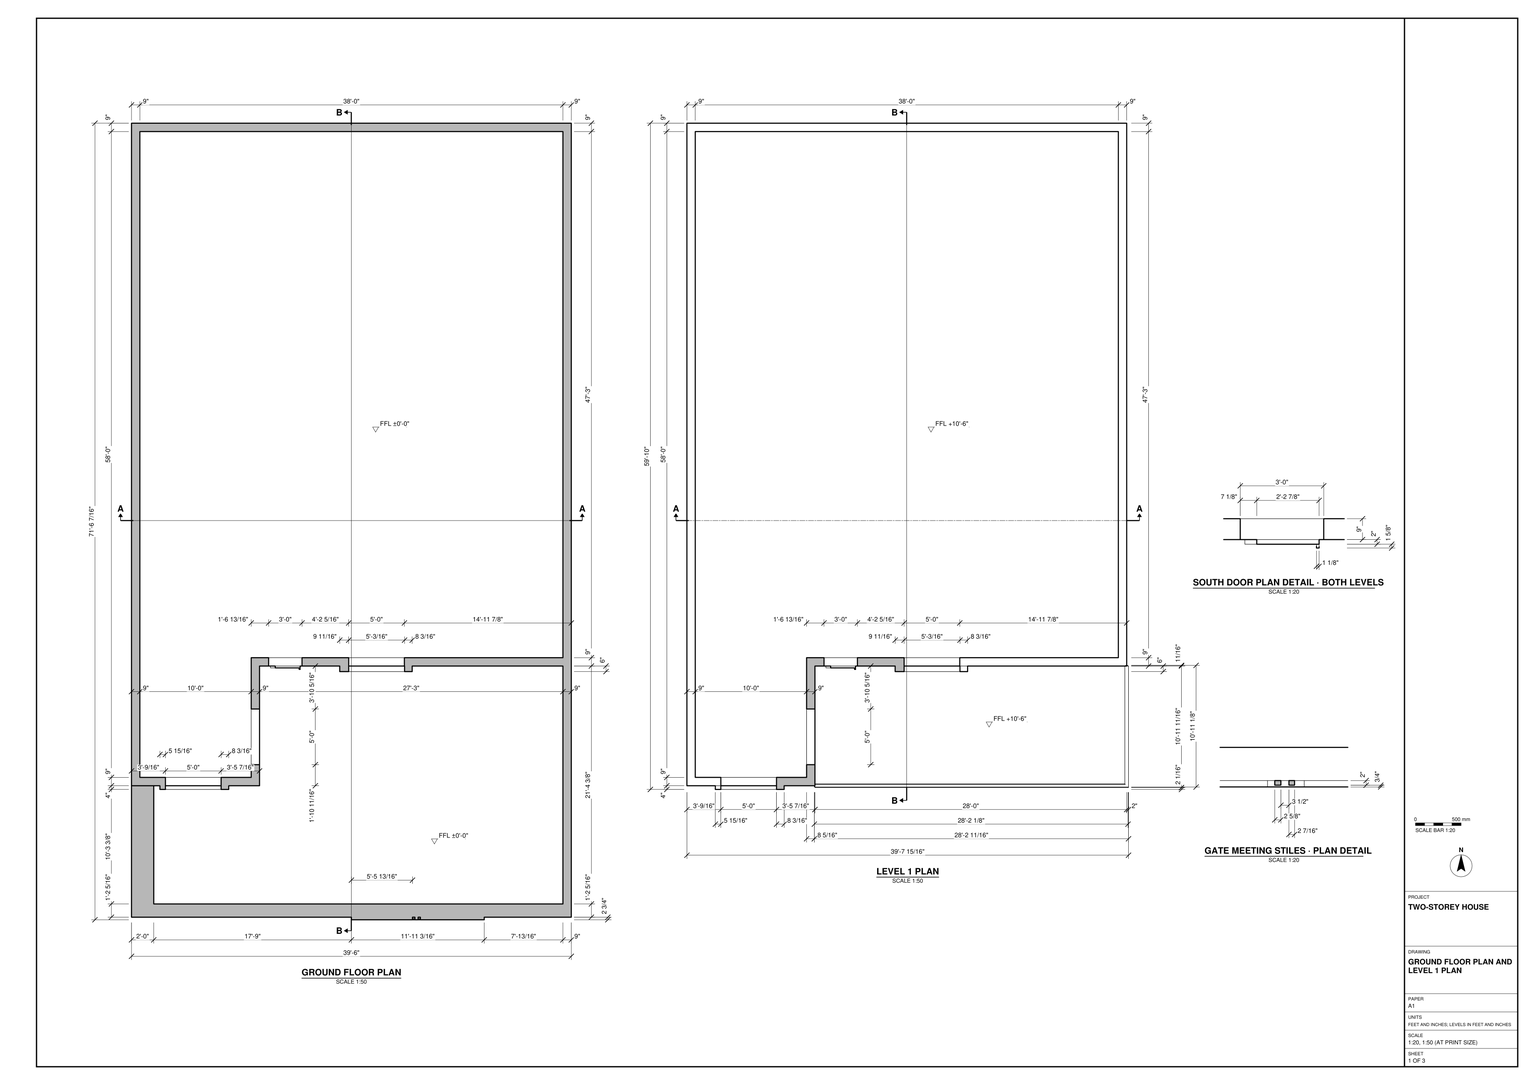
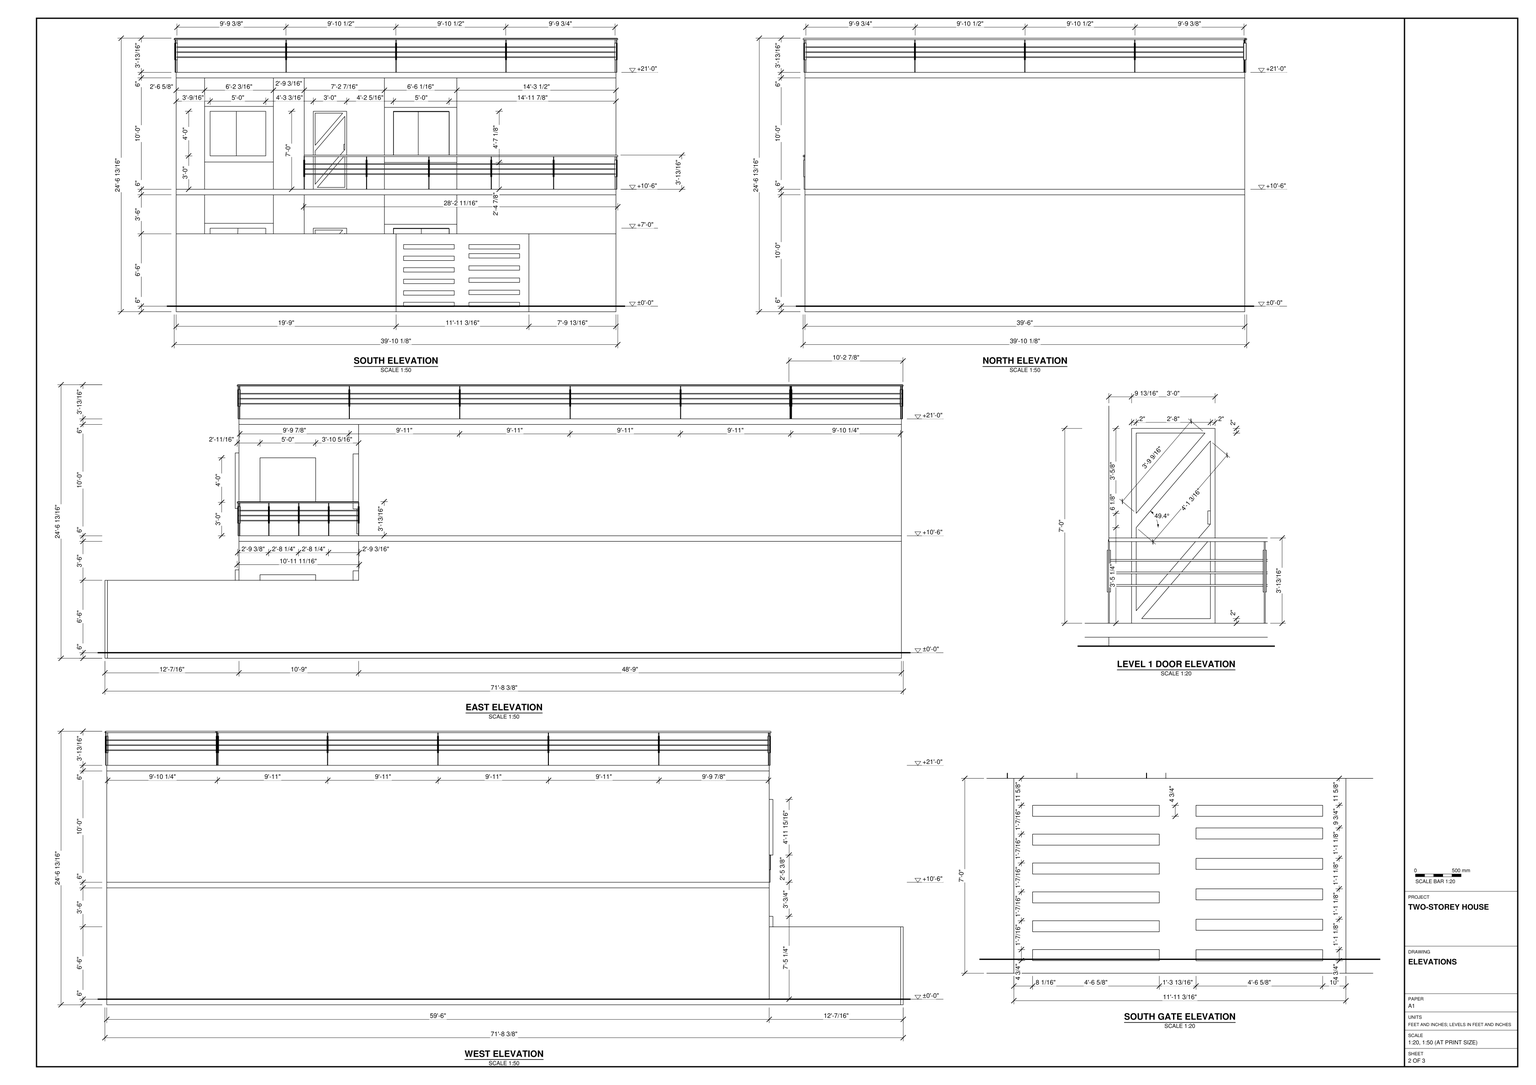
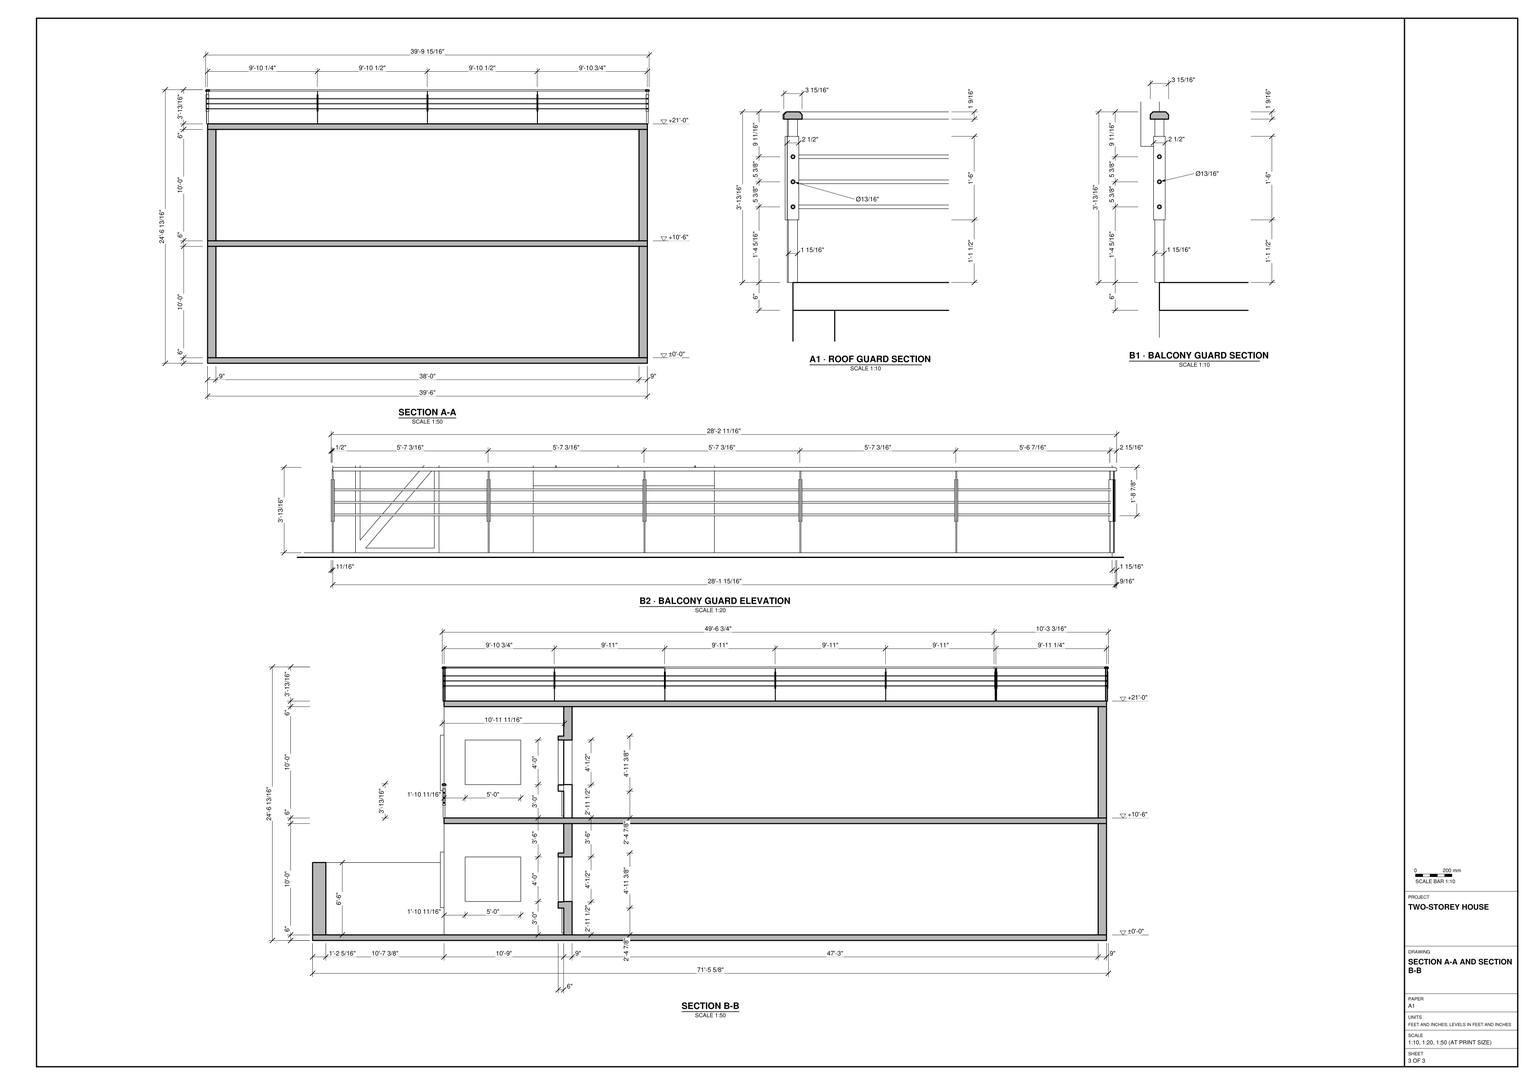
Build the house shown in task_files/diagram_01.pdf in SketchUp. Work in feet and inches. The overall model is 39'-10 3/16" wide from east to west, 71'-8 3/8" long from north to south and 24'-6 13/16" high. Set the finished floor levels at ±0'-0" and +10'-6".

Use the plans to lay out the open interior and the stepped south frontage. The west bay projects toward the forecourt, while the recessed wall beside it contains a door and a window on each floor. Follow the drawn wall thicknesses, including the 9" house walls. Use the sections to locate the ground slab, upper slab and flat roof. Extend the upper slab across the recess to form the balcony, with the roof continuing over it. Model the front and side runs of the balcony guard and the guard around the roof. Follow the details for the upper door, guard rails and posts, and the paired gate in the south forecourt wall.

Keep walls, slabs, roof, guards, gate and each furniture or joinery piece separate as groups or components. Use components for repeated parts. Any decor or loose items may be suitable library components. Save one SketchUp model as output_files/two_storey_house_with_a_balcony_and_gated_forecourt.skp.

# SketchUp Ruby script. Lengths in inches.
U = 1.inch
M = Sketchup.active_model
def pt(a) = Geom::Point3d.new(a.map { |v| v * U })
def face(e, loops, mat)
  f = e.add_face(loops[0].map { |a| pt(a) })
  loops[1..].each { |l| e.add_face(l.map { |a| pt(a) }).erase! }
  f.material = f.back_material = mat if mat
  f
end
# faces: each face lists its corners as indices into pts; further lists are holes
def faces(e, pts, list, mat = nil) = list.each { |f| face(e, (f[0].is_a?(Array) ? f : [f]).map { |l| l.map { |i| pts[i] } }, mat) }
# xy, xz, yz: faces in a plane at the given z, y or x. An outline is a flat list of corners, or four numbers for a rectangle; further outlines are holes
def ring(l) = l.size == 4 ? [[l[0], l[1]], [l[2], l[1]], [l[2], l[3]], [l[0], l[3]]] : l.each_slice(2).to_a
def flat(e, list, mat, &to3) = list.each { |f| face(e, (f[0].is_a?(Array) ? f : [f]).map { |l| ring(l).map { |u, v| to3.(u, v) } }, mat) }
def xy(e, z, list, mat = nil) = flat(e, list, mat) { |x, y| [x, y, z] }
def xz(e, y, list, mat = nil) = flat(e, list, mat) { |x, z| [x, y, z] }
def yz(e, x, list, mat = nil) = flat(e, list, mat) { |y, z| [x, y, z] }
def lines(e, pts, list) = list.each { |a, b| e.add_line(pt(pts[a]), pt(pts[b])) }
# prism: a flat outline (further loops are holes) pulled along v
def prism(e, loops, v, mat = nil)
  f = face(e, loops, mat); d = Geom::Vector3d.new(v.map { |x| x * U })
  f.pushpull(f.normal.samedirection?(d) ? d.length : -d.length)
end
def box(e, o, s, mat = nil) = prism(e, [[o, [o[0] + s[0], o[1], o[2]], [o[0] + s[0], o[1] + s[1], o[2]], [o[0], o[1] + s[1], o[2]]]], [0, 0, s[2]], mat)
def at(x, y, z, deg = 0) = Geom::Transformation.translation(pt([x, y, z])) * Geom::Transformation.rotation(ORIGIN, Z_AXIS, deg.degrees)
def axes(o, x, y, z) = Geom::Transformation.new([*x, 0, *y, 0, *z, 0, *pt(o).to_a, 1])
def part(name) = M.definitions.add(name)
# library, detail: a bought-in or finely detailed component or shape, given as its bounding box
def library(name, o, s) = part(name).tap { |d| box(d.entities, o, s) }
def detail(e, o, s) = box(e.add_group.entities, o, s)
def put(e, d, t, mat = nil) = e.add_instance(d, t).tap { |i| i.material = mat if mat }
def group(e, t, mat = nil) = e.add_group.tap { |g| g.transformation = t; g.material = mat if mat }.entities
root = M.entities
M.materials.add("Teddy_Bracelet").color = [145, 141, 147]
M.materials.add("Teddy_Shoes").color = [189, 191, 193]
M.materials.add("[Color H05]").color = [0, 255, 255]
M.materials.add("[Color M09]").color = [0, 0, 0]
M.materials.add("[Field Square Tile]").color = [217, 201, 169]
M.materials.add("[Herringbone]").color = [130, 130, 130]
M.materials.add("[Translucent Glass Blue]").color = [100, 149, 237]
M.materials["[Translucent Glass Blue]"].alpha = 0.5
M.materials.add("[Wood Board Cork]").color = [215, 201, 115]
M.materials.add("[Wood Cherry Original]").color = [152, 86, 42]
M.materials.add("[Wood Veneer 02]").color = [190, 128, 91]
c1 = part("Ploe\#6")
box(c1.entities,[996.33,35.02,126],[0.47,1.96,36])
box(c1.entities,[996.8,34.74,139.5],[0.47,2.52,18],"[Wood Veneer 02]")
box(c1.entities,[995.85,34.74,139.5],[0.48,2.52,18],"[Wood Veneer 02]")
c2 = part("Group59\#1")
put(c2.entities,c1,at(0,0,0))
put(c2.entities,c1,at(2060.32,72,0,-180))
put(c2.entities,c1,at(134.4,0,0))
put(c2.entities,c1,at(2194.72,72,0,180))
put(c2.entities,c1,at(268.8,0,0))
put(c2.entities,c1,at(653.34,-694.13,0,45))
put(c2.entities,c1,at(1368.5625,-928.3125,0,90))
put(c2.entities,c1,at(1296.5625,1097.0625,0,-90))
put(c2.entities,c1,at(1368.5625,-863.8125,0,90))
put(c2.entities,c1,at(1296.5625,1161.5625,0,-90))
c3 = library("Group\#8",[0,0,0],[337.97,130.97,20.87])
c4 = part("Ploe\#4")
box(c4.entities,[858.33,749.02,252],[0.47,1.96,36])
box(c4.entities,[858.8,748.74,265.5],[0.47,2.52,18],"[Wood Veneer 02]")
box(c4.entities,[857.85,748.74,265.5],[0.48,2.52,18],"[Wood Veneer 02]")
c5 = part("Group51\#1")
put(c5.entities,c4,at(0,0,0))
put(c5.entities,c4,at(1835.625,1500,0,180))
put(c5.entities,c4,at(237,0,0))
put(c5.entities,c4,at(2072.625,1500,0,180))
put(c5.entities,c4,at(195.14,826.77,0,-45))
put(c5.entities,c4,at(2082.5625,-227.5625,0,90))
put(c5.entities,c4,at(582.5625,1370.5625,0,-90))
put(c5.entities,c4,at(2082.5625,-465.5625,0,90))
put(c5.entities,c4,at(582.5625,1132.5625,0,-90))
put(c5.entities,c4,at(2082.5625,-703.5625,0,90))
put(c5.entities,c4,at(1409.33,1173.43,0,-135))
put(c5.entities,c4,at(355.5,-714,0))
put(c5.entities,c4,at(1954.125,786,0,180))
put(c5.entities,c4,at(118.5,-714,0))
put(c5.entities,c4,at(1995.99,-40.77,0,135))
put(c5.entities,c4,at(108.5625,1013.5625,0,-90))
put(c5.entities,c4,at(1608.5625,-584.5625,0,90))
put(c5.entities,c4,at(108.5625,1251.5625,0,-90))
put(c5.entities,c4,at(1608.5625,-346.5625,0,90))
put(c5.entities,c4,at(108.5625,1489.5625,0,-90))
c6 = library("Group\#4",[0,0,0],[477.9375,717.9375,20.87])
c7 = library("Group\#7",[0,0,0],[3.9375,122.9,36.79])
xy(root,0,[[304.23,0.75,306.86,2.75],[310.33,0.75,312.76,2.75]],"[Color M09]")
xy(root,65.32,[[310.33,0.75,312.76,2.75]],"[Color M09]")
xy(root,65.54,[[304.23,0.75,306.86,2.75]],"[Color M09]")
xz(root,0.75,[[304.23,0,306.86,65.54],[310.33,0,312.76,65.32]],"[Color M09]")
xz(root,2.75,[[304.23,0,306.86,65.54],[310.33,0,312.76,65.32]])
yz(root,304.23,[[0.75,0,2.75,65.54]],"[Color M09]")
yz(root,306.86,[[0.75,0,2.75,65.54]],"[Color M09]")
yz(root,310.33,[[0.75,0,2.75,65.32]],"[Color M09]")
yz(root,312.76,[[0.75,0,2.75,65.32]],"[Color M09]")
g1 = group(root,at(1.39,144.4375,0),"[Herringbone]")
xy(g1,-6,[[237,-144.4375,372.91,-141.6875],[372.91,-144.4375,380.16,-141.6875]])
xy(g1,-0.62,[[315.52,-144.4375,370.15,-141.6875]])
xy(g1,-0.56,[[245.09,-144.4375,299.71,-141.6875]])
xy(g1,0,[[96.57,0,96.57,9,129,9,129,82.7,138,82.7,138,0],[147.78,129,183.78,138],[183.78,129,294.1,138]])
xy(g1,0,[[24,-127.39,465,-127.39,465,129,138,129,138,0,24,0]],"[Field Square Tile]")
xy(g1,2,[[152.13,127,181.79,129]])
xy(g1,4.13,[[315.52,-144.4375,370.15,-141.6875]])
xy(g1,4.19,[[245.09,-144.4375,299.71,-141.6875]])
xy(g1,11.88,[[245.09,-144.4375,299.71,-141.6875]])
xy(g1,12.51,[[315.52,-144.4375,370.15,-141.6875]])
xy(g1,16.63,[[245.09,-144.4375,299.71,-141.6875]])
xy(g1,17.26,[[315.52,-144.4375,370.15,-141.6875]])
xy(g1,24.32,[[245.09,-144.4375,299.71,-141.6875]])
xy(g1,25.63,[[315.52,-144.4375,370.15,-141.6875]])
xy(g1,28.875,[[224.4375,123,228.36,129],[228.36,123,302.52,129]],"Teddy_Bracelet")
xy(g1,29.07,[[245.09,-144.4375,299.71,-141.6875]])
xy(g1,29.35,[[30.625,-4,104.79,0]],"Teddy_Bracelet")
xy(g1,30.38,[[315.52,-144.4375,370.15,-141.6875]])
xy(g1,35.53,[[234.3,123,294.3,129]])
xy(g1,36,[[36.57,0,96.57,9],[129,22.7,138,82.7],[234.1,123,234.3,129],[234.1,129,294.1,138]])
xy(g1,36,[[36.57,-4,96.57,0]],"Teddy_Bracelet")
xy(g1,36.76,[[245.09,-144.4375,299.71,-141.6875]])
xy(g1,38.76,[[315.52,-144.4375,370.15,-141.6875]])
xy(g1,41.51,[[245.09,-144.4375,299.71,-141.6875]])
xy(g1,42.74,[[180.65,125.375,181.79,127]])
xy(g1,43.51,[[315.52,-144.4375,370.15,-141.6875]])
xy(g1,48.45,[[180.65,125.375,181.79,127]],"[Wood Cherry Original]")
xy(g1,49.19,[[245.09,-144.4375,299.71,-141.6875]])
xy(g1,51.88,[[315.52,-144.4375,370.15,-141.6875]])
xy(g1,53.94,[[245.09,-144.4375,299.71,-141.6875]])
xy(g1,56.63,[[315.52,-144.4375,370.15,-141.6875]])
xy(g1,61.63,[[245.09,-144.4375,299.71,-141.6875],[315.52,-144.4375,370.15,-141.6875]])
xy(g1,66.38,[[245.09,-144.4375,299.71,-141.6875],[315.52,-144.4375,370.15,-141.6875]])
xy(g1,78,[[237,-144.4375,380.16,-144.4375,380.16,-141.6875,474,-141.6875,474,129,465,129,465,-127.39,24,-127.39,24,0,0,0,0,-141.6875,237,-141.6875]])
xy(g1,82,[[149.78,127,179.4375,129]],"[Wood Cherry Original]")
xy(g1,83.53,[[294.1,123,294.3,129]])
xy(g1,84,[[36.57,0,96.57,9],[129,22.7,138,82.7],[147.78,129,183.78,138],[234.1,129,294.1,138]])
xy(g1,84,[[36.57,-4,96.57,0]],"Teddy_Bracelet")
xy(g1,84,[[234.1,123,294.1,129]],"Teddy_Shoes")
xy(g1,88.23,[[224.4375,123,302.52,129]],"Teddy_Shoes")
xy(g1,89.26,[[30.625,-4,104.79,0]],"Teddy_Bracelet")
xy(g1,120,[[[0,0,138,0,138,129,474,129,474,714,0,714],[9,9,9,705,465,705,465,138,129,138,129,9]]])
xy(g1,126,[[0,0,0,714,474,714,474,129,294.1,129,294.1,138,465,138,465,705,9,705,9,9,96.57,9,96.57,0],[96.57,0,96.57,9,129,9,129,82.7,138,82.7,138,0],[147.78,129,183.78,138],[183.78,129,294.1,138]])
xy(g1,128,[[152.13,127,181.79,129]])
xy(g1,154.875,[[224.4375,123,228.36,129],[228.36,123,302.52,129]],"Teddy_Bracelet")
xy(g1,155.35,[[30.625,-4,104.79,0]],"Teddy_Bracelet")
xy(g1,161.53,[[234.3,123,294.3,129]])
xy(g1,162,[[36.57,0,96.57,9],[129,22.7,138,82.7],[234.1,123,234.3,129],[234.1,129,294.1,138]])
xy(g1,162,[[36.57,-4,96.57,0]],"Teddy_Bracelet")
xy(g1,168.74,[[180.65,125.375,181.79,127]])
xy(g1,174.45,[[180.65,125.375,181.79,127]],"[Wood Cherry Original]")
xy(g1,208,[[149.78,127,179.4375,129]],"[Wood Cherry Original]")
xy(g1,209.53,[[294.1,123,294.3,129]])
xy(g1,210,[[36.57,0,96.57,9],[129,22.7,138,82.7],[147.78,129,183.78,138],[234.1,129,294.1,138]])
xy(g1,210,[[36.57,-4,96.57,0]],"Teddy_Bracelet")
xy(g1,210,[[234.1,123,294.1,129]],"Teddy_Shoes")
xy(g1,214.23,[[224.4375,123,302.52,129]],"Teddy_Shoes")
xy(g1,215.26,[[30.625,-4,104.79,0]],"Teddy_Bracelet")
xy(g1,246,[[[0,0,138,0,138,129,474,129,474,714,0,714],[9,9,9,705,465,705,465,138,129,138,129,9]]])
xz(g1,-144.4375,[[[237,-6,380.16,78],[315.52,-0.62,370.15,4.13],[315.52,12.51,370.15,17.26],[315.52,25.63,370.15,30.38],[315.52,38.76,370.15,43.51],[245.09,-0.56,299.71,4.19],[315.52,61.63,370.15,66.38],[315.52,51.88,370.15,56.63],[245.09,11.88,299.71,16.63],[245.09,36.76,299.71,41.51],[245.09,24.32,299.71,29.07],[245.09,61.63,299.71,66.38],[245.09,49.19,299.71,53.94]]])
xz(g1,-141.6875,[[315.52,-0.62,370.15,0],[245.09,-0.56,299.71,0],[0,0,237,78],[380.16,0,474,78],[245.09,36.76,299.71,41.51],
  [245.09,49.19,299.71,53.94],[245.09,61.63,299.71,66.38]])
xz(g1,-141.6875,[[245.09,0,299.71,4.19],[315.52,0,370.15,4.13],[245.09,11.88,299.71,16.63],[315.52,12.51,370.15,17.26],[245.09,24.32,299.71,29.07],
  [315.52,25.63,370.15,30.38],[315.52,38.76,370.15,43.51],[315.52,51.88,370.15,56.63]],"[Color H05]")
xz(g1,-127.39,[[24,0,465,78]],"[Color H05]")
xz(g1,-4,[[[30.625,29.35,104.79,89.26],[36.57,36,96.57,84]],[[30.625,155.35,104.79,215.26],[36.57,162,96.57,210]]],"Teddy_Shoes")
xz(g1,0,[[24,0,30.625,0,30.625,120,0,120,0,78,24,78],[9,0,24,78],[30.625,0,104.79,29.35],[104.79,0,138,120],[30.625,89.26,104.79,120],
  [0,126,30.625,246],[30.625,126,104.79,155.35],[104.79,126,138,246],[30.625,215.26,104.79,246]])
xz(g1,0,[[36.57,36,64.85,36,66.57,84,36.57,84],[64.85,36,96.57,36,96.57,84,66.57,84],[36.57,162,64.85,210],[64.85,162,96.57,210]],"[Translucent Glass Blue]")
xz(g1,9,[[[9,0,129,120],[36.57,36,96.57,84]],[[9,126,129,246],[36.57,162,96.57,210]]])
xz(g1,22.7,[[129,36,138,84],[129,162,138,210]])
xz(g1,82.7,[[129,36,138,84],[129,162,138,210]])
xz(g1,123,[[[224.4375,28.875,302.52,88.23],[234.3,35.53,234.3,36,234.1,36,234.1,84,294.1,84,294.1,83.53,294.3,83.53,294.3,35.53]],[[224.4375,154.875,302.52,214.23],[234.3,161.53,234.3,162,234.1,162,234.1,210,294.1,210,294.1,209.53,294.3,209.53,294.3,161.53]]],"Teddy_Shoes")
xz(g1,125.375,[[180.65,42.74,181.79,48.45],[180.65,168.74,181.79,174.45]],"[Wood Cherry Original]")
xz(g1,127,[[180.65,42.74,181.79,48.45],[180.65,168.74,181.79,174.45]])
xz(g1,127,[[152.13,2,181.79,2,181.79,36.59],[149.78,5.41,181.79,42.74,180.65,42.74,180.65,48.45,181.79,48.45,181.79,78.59,149.78,41.26],[149.78,47.41,179.4375,82,149.78,82],[152.13,128,181.79,128,181.79,162.59],[149.78,131.41,181.79,168.74,180.65,168.74,180.65,174.45,181.79,174.45,181.79,204.59,149.78,167.26],
  [149.78,173.41,179.4375,208,149.78,208]],"[Wood Board Cork]")
xz(g1,129,[[138,0,147.78,0,147.78,84,183.78,84,183.78,0,224.4375,0,224.4375,120,138,120],[224.4375,0,302.52,28.875],[302.52,0,465,0,465,78,474,78,474,120,302.52,120],[234.3,35.53,264.2,36],[264.2,35.53,294.3,35.53,294.3,83.53,294.1,83.53,294.1,36,264.2,36],
  [224.4375,88.23,302.52,120],[138,126,147.78,126,147.78,210,183.78,210,183.78,126,224.4375,126,224.4375,246,138,246],[224.4375,126,302.52,154.875],[302.52,126,474,246],[224.4375,214.23,302.52,246]])
xz(g1,129,[[234.1,36,234.3,36,234.3,83.53,294.1,83.53,294.1,84,234.1,84],[234.3,36,264.2,83.53],[264.2,36,294.1,83.53],[234.1,162,234.3,162,234.3,209.53,294.1,209.53,294.1,210,234.1,210],[234.3,162,260.9375,209.53],
  [260.9375,162,294.1,209.53]],"[Translucent Glass Blue]")
xz(g1,129,[[[147.78,0,183.78,84],[149.78,5.41,149.78,41.26,181.79,78.59,181.79,42.74],[152.13,2,181.79,36.59,181.79,2],[149.78,47.41,149.78,82,179.4375,82]],[[147.78,126,183.78,210],[149.78,131.41,149.78,167.26,181.79,204.59,181.79,168.74],[152.13,128,181.79,162.59,181.79,128],[149.78,173.41,149.78,208,179.4375,208]]],"[Wood Cherry Original]")
xz(g1,138,[[[129,0,129,120,465,120,465,0,183.78,0,183.78,84,147.78,84,147.78,0],[234.1,36,294.1,84]],[[129,126,129,246,465,246,465,126,183.78,126,183.78,210,147.78,210,147.78,126],[234.1,162,294.1,210]]])
xz(g1,705,[[9,0,465,120],[9,126,465,246]])
xz(g1,714,[[0,0,474,120],[0,126,474,246]])
yz(g1,0,[[-141.6875,0,0,78],[0,0,714,120],[0,126,714,246]])
yz(g1,9,[[9,0,705,120],[9,126,705,246]])
yz(g1,24,[[-127.39,0,0,78]])
yz(g1,30.625,[[-4,29.35,0,89.26],[-4,155.35,0,215.26]],"Teddy_Bracelet")
yz(g1,36.57,[[0,36,9,84],[0,162,9,210]])
yz(g1,36.57,[[-4,36,0,84],[-4,162,0,210]],"Teddy_Bracelet")
yz(g1,96.57,[[0,36,9,84],[0,162,9,210]])
yz(g1,96.57,[[-4,36,0,84],[-4,162,0,210]],"Teddy_Bracelet")
yz(g1,104.79,[[-4,29.35,0,89.26],[-4,155.35,0,215.26]],"Teddy_Bracelet")
yz(g1,129,[[[9,0,138,120],[22.7,36,82.7,84]],[[9,126,138,246],[22.7,162,82.7,210]]])
yz(g1,138,[[[0,0,129,120],[22.7,36,82.7,84]],[[0,126,129,246],[22.7,162,82.7,210]]])
yz(g1,138,[[22.7,36,82.7,84],[22.7,162,82.7,210]],"[Translucent Glass Blue]")
yz(g1,147.78,[[129,0,138,84],[129,126,138,210]])
yz(g1,149.78,[[127,5.41,129,41.26],[127,47.41,129,82],[127,131.41,129,167.26],[127,173.41,129,208]])
yz(g1,180.65,[[125.375,42.74,125.375,48.45,127,48.45,127,47.34,126.125,47.34,126.125,44.09,127,44.09,127,42.74],[125.375,168.74,125.375,174.45,127,174.45,127,173.34,126.125,173.34,126.125,170.09,127,170.09,127,168.74]],"[Wood Cherry Original]")
yz(g1,181.79,[[127,2,129,36.59],[127,42.74,129,78.59],[127,128,129,162.59],[127,168.74,129,204.59]])
yz(g1,181.79,[[125.375,42.74,127,42.74,127,43.57,125.9375,43.57,125.9375,47.44,127,47.44,127,48.45,125.375,48.45],[125.375,168.74,127,168.74,127,169.57,125.9375,169.57,125.9375,173.44,127,173.44,127,174.45,125.375,174.45]],"[Wood Cherry Original]")
yz(g1,183.78,[[129,0,138,84],[129,126,138,210]])
yz(g1,224.4375,[[123,28.875,129,88.23],[123,154.875,129,214.23]],"Teddy_Shoes")
yz(g1,234.1,[[129,36,138,84],[129,162,138,210]])
yz(g1,234.1,[[123,36,129,84],[123,162,129,210]],"Teddy_Shoes")
yz(g1,234.3,[[123,35.53,129,36],[123,161.53,129,162]])
yz(g1,237,[[-144.4375,-6,-141.6875,0],[-144.4375,0,-141.6875,78]])
yz(g1,245.09,[[-144.4375,-0.56,-141.6875,0],[-144.4375,0,-141.6875,4.19],[-144.4375,11.88,-141.6875,16.63],[-144.4375,24.32,-141.6875,29.07],[-144.4375,36.76,-141.6875,41.51],
  [-144.4375,49.19,-141.6875,53.94],[-144.4375,61.63,-141.6875,66.38]])
yz(g1,294.1,[[129,36,138,84],[123,83.53,129,84],[129,162,138,210],[123,209.53,129,210]])
yz(g1,294.3,[[123,35.53,129,83.53],[123,161.53,129,209.53]],"Teddy_Shoes")
yz(g1,299.71,[[-144.4375,-0.56,-141.6875,0],[-144.4375,0,-141.6875,4.19],[-144.4375,11.88,-141.6875,16.63],[-144.4375,24.32,-141.6875,29.07],[-144.4375,36.76,-141.6875,41.51],
  [-144.4375,49.19,-141.6875,53.94],[-144.4375,61.63,-141.6875,66.38]])
yz(g1,302.52,[[123,28.875,129,88.23],[123,154.875,129,214.23]],"Teddy_Shoes")
yz(g1,315.52,[[-144.4375,-0.62,-141.6875,0],[-144.4375,0,-141.6875,4.13],[-144.4375,12.51,-141.6875,17.26],[-144.4375,25.63,-141.6875,30.38],[-144.4375,38.76,-141.6875,43.51],
  [-144.4375,51.88,-141.6875,56.63],[-144.4375,61.63,-141.6875,66.38]])
yz(g1,370.15,[[-144.4375,-0.62,-141.6875,0],[-144.4375,0,-141.6875,4.13],[-144.4375,12.51,-141.6875,17.26],[-144.4375,25.63,-141.6875,30.38],[-144.4375,38.76,-141.6875,43.51],
  [-144.4375,51.88,-141.6875,56.63],[-144.4375,61.63,-141.6875,66.38]])
yz(g1,380.16,[[-144.4375,-6,-141.6875,0],[-144.4375,0,-141.6875,78]])
yz(g1,465,[[-127.39,0,129,78],[138,0,705,120],[138,126,705,246]])
yz(g1,474,[[-141.6875,0,714,0,714,120,129,120,129,78,-141.6875,78],[129,126,714,246]])
p = [[181.79,129,36.59],[152.13,129,2],[152.13,127,2],[181.79,127,36.59],[149.78,129,5.41],[181.79,129,42.74],
  [181.79,127,42.74],[149.78,127,5.41],[181.79,129,78.59],[149.78,129,41.26],[149.78,127,41.26],[181.79,127,78.59],
  [149.78,129,47.41],[179.4375,129,82],[179.4375,127,82],[149.78,127,47.41],[181.79,129,162.59],[152.13,129,128],
  [152.13,127,128],[181.79,127,162.59],[149.78,129,131.41],[181.79,129,168.74],[181.79,127,168.74],[149.78,127,131.41],
  [181.79,129,204.59],[149.78,129,167.26],[149.78,127,167.26],[181.79,127,204.59],[149.78,129,173.41],[179.4375,129,208],
  [179.4375,127,208],[149.78,127,173.41],[138,0,126],[474,0,126],[474,-27,-6],[474,-27.1875,-6],
  [465,-27,-6],[465,129,-6],[474,129,-6],[465,-27.1875,-6],[465,-127.39,0],[465,-141.6875,0],
  [237,-141.6875,0],[245.09,-141.6875,0],[299.71,-141.6875,0],[315.52,-141.6875,0],[370.15,-141.6875,0],[380.16,-141.6875,0],
  [0,-27,-6],[0,-35.1875,-6],[9,-27,-6],[9,0,-6],[0,0,-6]]
faces(g1,p,[[0,1,2,3],[4,5,6,7],[8,9,10,11],[12,13,14,15],[16,17,18,19],[20,21,22,23],[24,25,26,27],[28,29,30,31]])
lines(g1,p,[[32,33],[34,35],[36,37],[34,36],[38,34],[39,36],[40,41],[42,43],[44,45],[46,47],[48,49],[50,48],
  [50,51],[52,48]])
g2 = group(g1,at(137.29,-1.97,126))
put(g2,c2,at(-995.85,-34.03,-126))
put(g2,c3,at(0.71,0,15.92))
g3 = group(g1,at(0,0,0),"[Field Square Tile]")
box(g3,[0,-141.6875,-6],[474,855.6875,6])
box(g3,[0,0,246],[474,714,6])
xy(g3,126,[[0,0,474,714]])
xz(g3,0,[[0,120,474,126]])
g4 = group(g3,at(-1.97,-1.97,252))
put(g4,c5,at(-856.59,-34.03,-252))
put(g4,c6,at(0,0,15.92))
put(g3,c7,at(-2.2,592.8,252))
g5 = group(g1,at(0,0,120))
xy(g5,0,[[0,0,474,714]])
xz(g5,714,[[0,0,474,6]])
yz(g5,0,[[0,0,714,6]])
yz(g5,474,[[0,0,714,6]])
g6 = group(g1,at(0,0,0))
xz(g6,0,[[0,0,9,78]])
